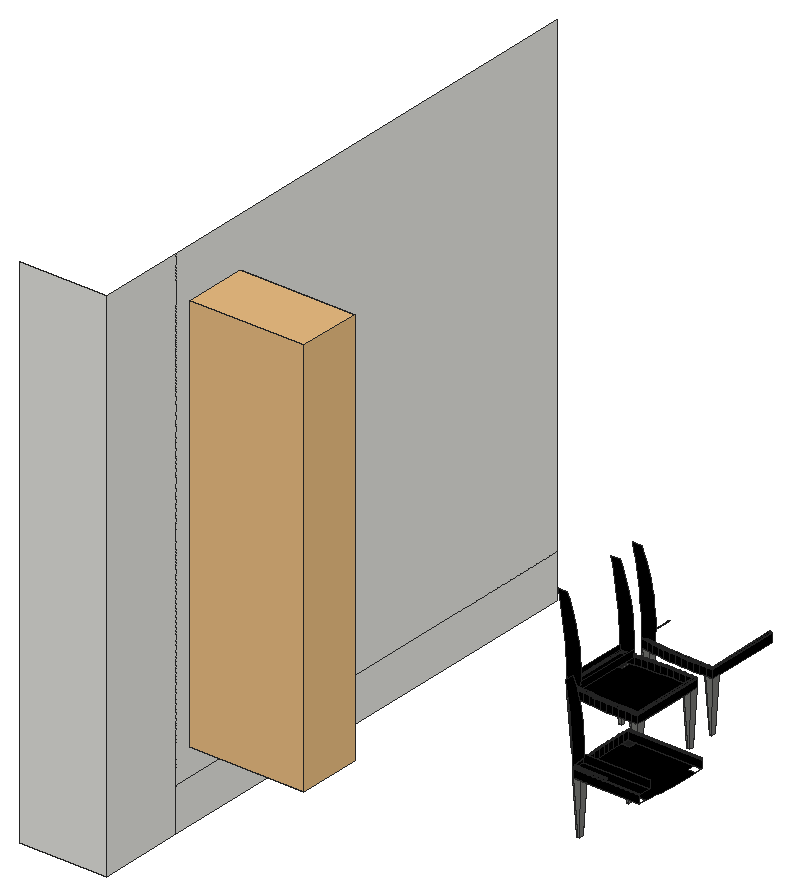
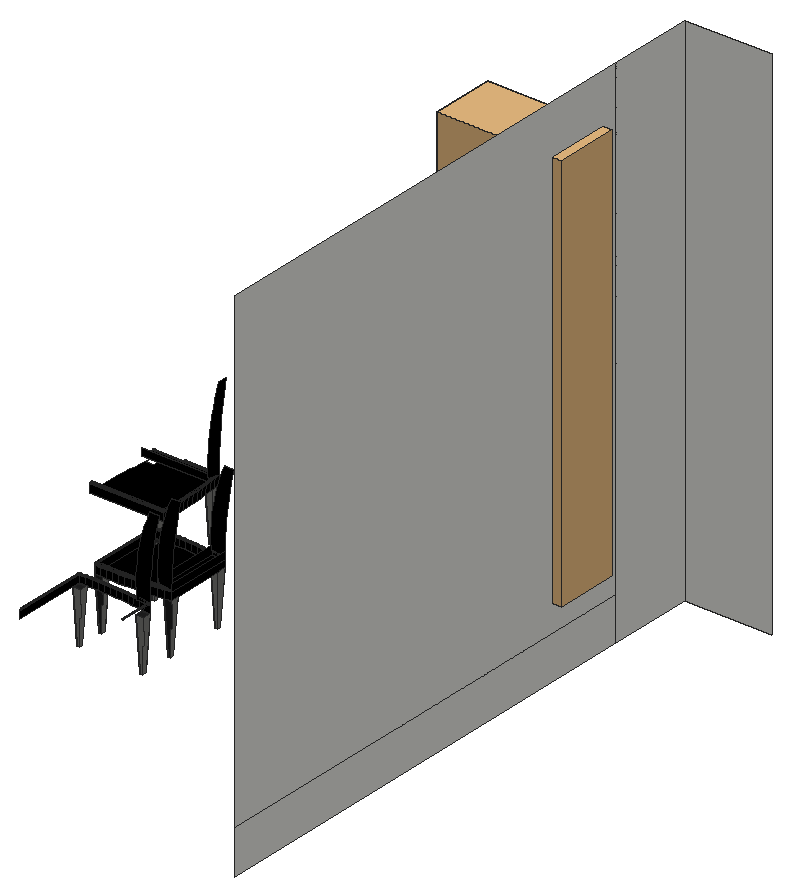
# SketchUp Ruby script. Lengths in inches.
U = 1.inch
M = Sketchup.active_model
def pt(a) = Geom::Point3d.new(a.map { |v| v * U })
def face(e, loops, mat)
  f = e.add_face(loops[0].map { |a| pt(a) })
  loops[1..].each { |l| e.add_face(l.map { |a| pt(a) }).erase! }
  f.material = f.back_material = mat if mat
  f
end
# faces: each face lists its corners as indices into pts; further lists are holes
def faces(e, pts, list, mat = nil) = list.each { |f| face(e, (f[0].is_a?(Array) ? f : [f]).map { |l| l.map { |i| pts[i] } }, mat) }
# xy, xz, yz: faces in a plane at the given z, y or x. An outline is a flat list of corners, or four numbers for a rectangle; further outlines are holes
def ring(l) = l.size == 4 ? [[l[0], l[1]], [l[2], l[1]], [l[2], l[3]], [l[0], l[3]]] : l.each_slice(2).to_a
def flat(e, list, mat, &to3) = list.each { |f| face(e, (f[0].is_a?(Array) ? f : [f]).map { |l| ring(l).map { |u, v| to3.(u, v) } }, mat) }
def xy(e, z, list, mat = nil) = flat(e, list, mat) { |x, y| [x, y, z] }
def xz(e, y, list, mat = nil) = flat(e, list, mat) { |x, z| [x, y, z] }
def yz(e, x, list, mat = nil) = flat(e, list, mat) { |y, z| [x, y, z] }
def lines(e, pts, list) = list.each { |a, b| e.add_line(pt(pts[a]), pt(pts[b])) }
# prism: a flat outline (further loops are holes) pulled along v
def prism(e, loops, v, mat = nil)
  f = face(e, loops, mat); d = Geom::Vector3d.new(v.map { |x| x * U })
  f.pushpull(f.normal.samedirection?(d) ? d.length : -d.length)
end
def box(e, o, s, mat = nil) = prism(e, [[o, [o[0] + s[0], o[1], o[2]], [o[0] + s[0], o[1] + s[1], o[2]], [o[0], o[1] + s[1], o[2]]]], [0, 0, s[2]], mat)
def at(x, y, z, deg = 0) = Geom::Transformation.translation(pt([x, y, z])) * Geom::Transformation.rotation(ORIGIN, Z_AXIS, deg.degrees)
def axes(o, x, y, z) = Geom::Transformation.new([*x, 0, *y, 0, *z, 0, *pt(o).to_a, 1])
def part(name) = M.definitions.add(name)
# library, detail: a bought-in or finely detailed component or shape, given as its bounding box
def library(name, o, s) = part(name).tap { |d| box(d.entities, o, s) }
def detail(e, o, s) = box(e.add_group.entities, o, s)
def put(e, d, t, mat = nil) = e.add_instance(d, t).tap { |i| i.material = mat if mat }
def group(e, t, mat = nil) = e.add_group.tap { |g| g.transformation = t; g.material = mat if mat }.entities
root = M.entities
M.materials.add("Color_008").color = [30, 30, 30]
M.materials.add("[Color M09]").color = [0, 0, 0]
M.materials.add("[Metal Seamed]").color = [118, 119, 115]
c1 = library("Group\#1",[0,0,0],[34.5,17.48,110.79])
xy(root,12,[[105.836,60.75,106.653,61.567],[104.815,79.026,105.632,79.843],[100.046,87.836,100.863,88.653],[81.769,88.857,82.586,89.674],[81.769,105.091,82.586,105.908],
  [100.046,106.112,100.863,106.929],[100.046,113.742,100.863,114.558],[81.769,114.763,82.586,115.58]],"Color_008")
xy(root,26.704,[[105.172,60.085,107.317,62.231],[104.151,78.362,106.296,80.507],[99.382,87.171,101.527,89.317],[81.105,88.193,83.25,90.338],[81.105,104.427,83.25,106.572],
  [99.382,105.448,101.527,107.593],[99.382,113.077,101.527,115.223],[81.105,114.098,83.25,116.244]],"Color_008")
xy(root,26.704,[[105.172,60.085,104.932,61.775,104.719,63.469,104.535,65.165,104.379,66.865,104.252,68.567,104.152,70.271,104.081,71.976,104.038,73.682,104.024,75.389,104.038,77.096,104.08,78.802,104.151,80.507,104.151,78.362,106.296,78.362,106.296,80.507,122.427,80.507,122.427,78.362,124.573,78.362,124.573,80.507,124.643,78.802,124.686,77.096,124.7,75.389,124.685,73.682,124.642,71.976,124.571,70.271,124.472,68.567,124.344,66.865,124.188,65.165,124.004,63.469,123.792,61.775,123.552,60.085,123.552,62.231,121.406,62.231,121.406,60.085,107.317,60.085,107.317,62.231,105.172,62.231],[96.409,87.045,94.702,87.059,92.996,87.102,91.291,87.173,89.587,87.272,87.885,87.4,86.185,87.556,84.488,87.74,82.795,87.952,81.105,88.193,83.25,88.193,83.25,90.338,81.105,90.338,81.105,104.427,83.25,104.427,83.25,106.572,81.105,106.572,82.795,106.8125,84.488,107.025,86.185,107.209,87.885,107.365,89.587,107.493,91.291,107.592,92.996,107.663,94.702,107.706,96.409,107.72,98.115,107.706,99.822,107.664,101.527,107.593,99.382,107.593,99.382,105.448,101.527,105.448,101.527,89.317,99.382,89.317,99.382,87.171,101.527,87.171,99.822,87.101,98.115,87.058]],"[Color M09]")
xy(root,28.845,[[105.172,60.085,123.552,63.622],[81.105,88.193,84.642,106.572]],"[Color M09]")
xz(root,0,[[0,0,24,144]])
xz(root,60.085,[[105.172,26.704,123.552,28.845]],"[Color M09]")
xz(root,80.507,[[104.151,26.704,124.573,28.845]],"[Color M09]")
xz(root,88.193,[[81.105,28.845,81.079,30.792,81.019,32.738,80.925,34.683,80.797,36.626,80.634,38.566,80.438,40.503,80.208,42.436,79.945,44.365,79.647,46.29,79.316,48.208,78.952,50.121,78.554,52.027,81.004,52.027,81.733,50.191,82.387,48.328,82.965,46.44,83.466,44.53,83.89,42.602,84.235,40.658,84.502,38.701,84.689,36.736,84.797,34.764,84.825,32.79,84.773,30.816,84.642,28.845]],"[Color M09]")
xz(root,106.572,[[81.105,28.845,84.642,28.845,84.773,30.816,84.825,32.79,84.797,34.764,84.689,36.736,84.502,38.701,84.235,40.658,83.89,42.602,83.466,44.53,82.965,46.44,82.387,48.328,81.733,50.191,81.004,52.027,78.554,52.027,78.952,50.121,79.316,48.208,79.647,46.29,79.945,44.365,80.208,42.436,80.438,40.503,80.634,38.566,80.797,36.626,80.925,34.683,81.019,32.738,81.079,30.792]],"[Color M09]")
xz(root,114.098,[[81.105,28.845,81.079,30.792,81.019,32.738,80.925,34.683,80.797,36.626,80.634,38.566,80.438,40.503,80.208,42.436,79.945,44.365,79.647,46.29,79.316,48.208,78.952,50.121,78.554,52.027,81.004,52.027,81.733,50.191,82.387,48.328,82.965,46.44,83.466,44.53,83.89,42.602,84.235,40.658,84.502,38.701,84.689,36.736,84.797,34.764,84.825,32.79,84.773,30.816,84.642,28.845]],"[Color M09]")
yz(root,24,[[0,0,24,144],[24,0,156,12],[24,12,156,144]])
yz(root,81.105,[[88.193,26.704,106.572,28.845]],"[Color M09]")
yz(root,101.527,[[87.171,26.704,107.593,28.845],[113.077,26.704,133.499,28.845]],"[Color M09]")
yz(root,105.172,[[60.085,28.845,63.622,28.845,63.754,30.816,63.806,32.79,63.777,34.764,63.67,36.736,63.482,38.701,63.216,40.658,62.87,42.602,62.446,44.53,61.945,46.44,61.367,48.328,60.713,50.191,59.985,52.027,57.534,52.027,57.932,50.121,58.297,48.208,58.628,46.29,58.925,44.365,59.189,42.436,59.419,40.503,59.615,38.566,59.777,36.626,59.905,34.683,59.999,32.738,60.059,30.792]],"[Color M09]")
p = [[106.653,60.75,12],[107.317,60.085,26.704],[105.172,60.085,26.704],[105.836,60.75,12],[105.172,62.231,26.704],[105.836,61.567,12],
  [106.653,61.567,12],[107.317,62.231,26.704],[105.632,79.026,12],[106.296,78.362,26.704],[104.151,78.362,26.704],[104.815,79.026,12],
  [104.151,80.507,26.704],[104.815,79.843,12],[105.632,79.843,12],[106.296,80.507,26.704],[100.863,87.836,12],[101.527,87.171,26.704],
  [99.382,87.171,26.704],[100.046,87.836,12],[99.382,89.317,26.704],[100.046,88.653,12],[100.863,88.653,12],[101.527,89.317,26.704],
  [82.586,88.857,12],[83.25,88.193,26.704],[81.105,88.193,26.704],[81.769,88.857,12],[81.105,90.338,26.704],[81.769,89.674,12],
  [82.586,89.674,12],[83.25,90.338,26.704],[82.586,105.091,12],[83.25,104.427,26.704],[81.105,104.427,26.704],[81.769,105.091,12],
  [81.105,106.572,26.704],[81.769,105.908,12],[82.586,105.908,12],[83.25,106.572,26.704],[100.863,106.112,12],[101.527,105.448,26.704],
  [99.382,105.448,26.704],[100.046,106.112,12],[99.382,107.593,26.704],[100.046,106.929,12],[100.863,106.929,12],[101.527,107.593,26.704],
  [100.863,113.742,12],[101.527,113.077,26.704],[99.382,113.077,26.704],[100.046,113.742,12],[99.382,115.223,26.704],[100.046,114.558,12],
  [100.863,114.558,12],[101.527,115.223,26.704],[82.586,114.763,12],[83.25,114.098,26.704],[81.105,114.098,26.704],[81.769,114.763,12],
  [81.105,116.244,26.704],[81.769,115.58,12],[82.586,115.58,12],[83.25,116.244,26.704],[104.932,61.775,28.845],[104.932,61.775,26.704],
  [105.172,60.085,28.845],[104.719,63.469,28.845],[104.719,63.469,26.704],[104.535,65.165,28.845],[104.535,65.165,26.704],[104.379,66.865,28.845],
  [104.379,66.865,26.704],[104.252,68.567,28.845],[104.252,68.567,26.704],[104.152,70.271,28.845],[104.152,70.271,26.704],[104.081,71.976,28.845],
  [104.081,71.976,26.704],[104.038,73.682,26.704],[104.038,73.682,28.845],[104.024,75.389,26.704],[104.024,75.389,28.845],[104.038,77.096,26.704],
  [104.038,77.096,28.845],[104.08,78.802,26.704],[104.08,78.802,28.845],[104.151,80.507,28.845],[94.702,87.059,26.704],[94.702,87.059,28.845],
  [96.409,87.045,28.845],[96.409,87.045,26.704],[98.115,87.058,28.845],[98.115,87.058,26.704],[92.996,87.102,26.704],[92.996,87.102,28.845],
  [91.291,87.173,28.845],[91.291,87.173,26.704],[99.822,87.101,28.845],[99.822,87.101,26.704],[101.527,87.171,28.845],[89.587,87.272,28.845],
  [89.587,87.272,26.704],[87.885,87.4,28.845],[87.885,87.4,26.704],[86.185,87.556,28.845],[86.185,87.556,26.704],[84.488,87.74,28.845],
  [84.488,87.74,26.704],[82.795,87.952,28.845],[82.795,87.952,26.704],[81.105,88.193,28.845],[82.795,106.8125,28.845],[82.795,106.8125,26.704],
  [81.105,106.572,28.845],[84.488,107.025,28.845],[84.488,107.025,26.704],[86.185,107.209,28.845],[86.185,107.209,26.704],[87.885,107.365,28.845],
  [87.885,107.365,26.704],[89.587,107.493,28.845],[89.587,107.493,26.704],[91.291,107.592,28.845],[91.291,107.592,26.704],[92.996,107.663,28.845],
  [92.996,107.663,26.704],[99.822,107.664,28.845],[99.822,107.664,26.704],[101.527,107.593,28.845],[94.702,107.706,26.704],[94.702,107.706,28.845],
  [96.409,107.72,26.704],[96.409,107.72,28.845],[98.115,107.706,26.704],[98.115,107.706,28.845],[92.996,113.008,26.704],[92.996,113.008,28.845],
  [91.291,113.079,28.845],[91.291,113.079,26.704],[94.702,112.965,28.845],[94.702,112.965,26.704],[96.409,112.95,28.845],[96.409,112.95,26.704],
  [98.115,112.964,28.845],[98.115,112.964,26.704],[99.822,113.007,28.845],[99.822,113.007,26.704],[101.527,113.077,28.845],[89.587,113.178,28.845],
  [89.587,113.178,26.704],[87.885,113.306,28.845],[87.885,113.306,26.704],[86.185,113.462,28.845],[86.185,113.462,26.704],[84.488,113.646,28.845],
  [84.488,113.646,26.704],[82.795,113.858,28.845],[82.795,113.858,26.704],[81.105,114.098,28.845],[104.941,61.777,28.992],[105.18,60.095,28.992],
  [123.552,60.085,28.845],[123.543,60.095,28.992],[104.729,63.47,28.992],[104.545,65.166,28.992],[105.172,63.754,30.816],[105.172,63.622,28.845],
  [123.552,63.622,28.845],[123.552,63.754,30.816],[104.389,66.866,28.992],[104.261,68.568,28.992],[104.162,70.271,28.992],[104.091,71.976,28.992],
  [104.048,73.683,28.992],[104.034,75.389,28.992],[104.048,77.096,28.992],[104.09,78.802,28.992],[104.16,80.498,28.992],[94.702,87.069,28.992],
  [96.409,87.054,28.992],[98.115,87.068,28.992],[92.996,87.111,28.992],[91.291,87.182,28.992],[99.821,87.11,28.992],[101.517,87.181,28.992],
  [89.587,87.282,28.992],[101.517,107.584,28.992],[87.886,87.409,28.992],[86.186,87.565,28.992],[84.489,87.749,28.992],[82.796,87.962,28.992],
  [81.115,88.201,28.992],[81.079,106.572,30.792],[81.079,88.193,30.792],[81.115,106.564,28.992],[84.773,106.572,30.816],[84.642,106.572,28.845],
  [84.642,88.193,28.845],[84.773,88.193,30.816],[82.796,106.803,28.992],[84.489,107.015,28.992],[86.186,107.199,28.992],[87.886,107.355,28.992],
  [89.587,107.483,28.992],[91.291,107.582,28.992],[92.996,107.653,28.992],[99.821,107.654,28.992],[94.702,107.696,28.992],[96.409,107.71,28.992],
  [98.115,107.697,28.992],[92.996,113.017,28.992],[91.291,113.088,28.992],[94.702,112.974,28.992],[96.409,112.96,28.992],[98.115,112.974,28.992],
  [99.821,113.016,28.992],[101.517,113.087,28.992],[89.587,113.1875,28.992],[101.517,133.49,28.992],[101.527,133.499,28.845],[87.886,113.315,28.992],
  [86.186,113.471,28.992],[84.489,113.655,28.992],[82.796,113.868,28.992],[81.115,114.107,28.992],[104.97,61.78,29.137],[105.205,60.124,29.137],
  [123.518,60.124,29.137],[114.362,60.124,29.137],[104.757,63.473,29.137],[104.573,65.169,29.137],[104.417,66.868,29.137],[104.29,68.57,29.137],
  [104.191,70.273,29.137],[104.119,71.978,29.137],[104.077,73.683,29.137],[104.0625,75.389,29.137],[104.076,77.095,29.137],[104.119,78.801,29.137],
  [104.188,80.469,29.137],[124.563,80.498,28.992],[124.536,80.469,29.137],[92.997,87.14,29.137],[91.292,87.211,29.137],[94.703,87.097,29.137],
  [96.409,87.083,29.137],[98.115,87.097,29.137],[99.82,87.139,29.137],[101.489,87.208,29.137],[89.589,87.31,29.137],[101.489,107.556,29.137],
  [87.888,87.438,29.137],[86.189,87.594,29.137],[84.493,87.778,29.137],[82.8,87.99,29.137],[81.143,88.226,29.137],[81.143,106.539,29.137],
  [81.143,97.382,29.137],[82.8,106.774,29.137],[84.493,106.987,29.137],[86.189,107.171,29.137],[87.888,107.327,29.137],[89.589,107.454,29.137],
  [91.292,107.554,29.137],[92.997,107.625,29.137],[94.703,107.667,29.137],[98.115,107.668,29.137],[99.82,107.626,29.137],[96.409,107.682,29.137],
  [92.997,113.046,29.137],[91.292,113.117,29.137],[94.703,113.003,29.137],[96.409,112.989,29.137],[98.115,113.003,29.137],[99.82,113.045,29.137],
  [101.489,113.114,29.137],[89.589,113.216,29.137],[101.489,133.462,29.137],[87.888,113.344,29.137],[86.189,113.5,29.137],[84.493,113.684,29.137],
  [82.8,113.896,29.137],[81.143,114.132,29.137],[105.017,61.787,29.276],[105.246,60.171,29.276],[114.362,60.171,29.276],[104.804,63.479,29.276],
  [104.62,65.174,29.276],[104.465,66.872,29.276],[104.337,68.573,29.276],[104.238,70.275,29.276],[104.167,71.98,29.276],[104.167,71.978,29.276],
  [104.124,73.684,29.276],[104.11,75.389,29.276],[104.124,77.094,29.276],[104.166,78.799,29.276],[104.233,80.422,29.276],[124.49,80.422,29.276],
  [92.999,87.187,29.276],[92.998,87.187,29.276],[91.295,87.258,29.276],[94.703,87.145,29.276],[96.409,87.13,29.276],[98.114,87.144,29.276],
  [99.819,87.186,29.276],[101.441,87.254,29.276],[89.592,87.358,29.276],[101.441,107.511,29.276],[87.892,87.485,29.276],[86.194,87.641,29.276],
  [84.498,87.825,29.276],[82.806,88.037,29.276],[81.191,88.267,29.276],[81.191,97.382,29.276],[81.191,106.498,29.276],[82.806,106.728,29.276],
  [84.498,106.94,29.276],[86.194,107.124,29.276],[87.892,107.279,29.276],[89.592,107.407,29.276],[91.295,107.506,29.276],[92.999,107.577,29.276],
  [92.998,107.577,29.276],[99.819,107.578,29.276],[94.703,107.62,29.276],[96.409,107.634,29.276],[98.114,107.62,29.276],[92.999,113.093,29.276],
  [92.998,113.093,29.276],[91.295,113.164,29.276],[94.703,113.05,29.276],[96.409,113.036,29.276],[98.114,113.05,29.276],[99.819,113.092,29.276],
  [101.441,113.16,29.276],[89.592,113.263,29.276],[101.441,133.417,29.276],[87.892,113.391,29.276],[86.194,113.547,29.276],[84.498,113.731,29.276],
  [82.806,113.943,29.276],[81.191,114.173,29.276],[81.191,123.288,29.276],[81.143,123.288,29.137],[105.081,61.795,29.408],[105.303,60.236,29.408],
  [114.362,60.236,29.408],[104.869,63.486,29.408],[104.685,65.181,29.408],[104.529,66.878,29.408],[104.402,68.577,29.408],[104.303,70.278,29.408],
  [104.232,71.98,29.408],[104.189,73.685,29.408],[104.232,71.982,29.408],[104.175,75.389,29.408],[104.189,77.093,29.408],[104.231,78.797,29.408],
  [104.296,80.356,29.408],[124.428,80.356,29.408],[93.002,87.252,29.408],[94.705,87.21,29.408],[96.409,87.195,29.408],[98.113,87.209,29.408],
  [99.817,87.251,29.408],[93,87.252,29.408],[91.298,87.323,29.408],[101.376,87.316,29.408],[89.597,87.423,29.408],[101.376,107.449,29.408],
  [87.897,87.55,29.408],[86.2,87.706,29.408],[84.506,87.89,29.408],[82.815,88.102,29.408],[81.256,88.323,29.408],[81.256,97.382,29.408],
  [81.256,106.441,29.408],[82.815,106.663,29.408],[84.506,106.875,29.408],[86.2,107.059,29.408],[87.897,107.215,29.408],[89.597,107.342,29.408],
  [91.298,107.441,29.408],[93,107.512,29.408],[99.817,107.513,29.408],[93.002,107.512,29.408],[94.705,107.555,29.408],[98.113,107.555,29.408],
  [96.409,107.569,29.408],[94.705,113.116,29.408],[96.409,113.101,29.408],[98.113,113.115,29.408],[93,113.158,29.408],[91.298,113.229,29.408],
  [93.002,113.158,29.408],[99.817,113.157,29.408],[101.376,113.222,29.408],[89.597,113.328,29.408],[101.376,133.354,29.408],[87.897,113.456,29.408],
  [86.2,113.612,29.408],[84.506,113.795,29.408],[82.815,114.007,29.408],[81.256,114.229,29.408],[81.256,123.288,29.408],[105.162,61.806,29.531],
  [105.374,60.318,29.531],[114.362,60.318,29.531],[104.95,63.496,29.531],[104.767,65.189,29.531],[104.611,66.884,29.531],[104.484,68.583,29.531],
  [104.384,70.283,29.531],[104.314,71.982,29.531],[104.313,71.986,29.531],[104.271,73.686,29.531],[104.257,75.389,29.531],[104.27,77.092,29.531],
  [104.313,78.794,29.531],[104.374,80.275,29.531],[124.35,80.275,29.531],[93.006,87.334,29.531],[94.706,87.291,29.531],[96.409,87.277,29.531],
  [98.112,87.291,29.531],[99.814,87.333,29.531],[91.302,87.405,29.531],[89.602,87.504,29.531],[93.002,87.334,29.531],[101.294,87.395,29.531],
  [101.294,107.37,29.531],[87.904,87.631,29.531],[86.208,87.787,29.531],[84.515,87.971,29.531],[82.826,88.183,29.531],[81.338,88.394,29.531],
  [81.338,97.382,29.531],[81.338,106.37,29.531],[82.826,106.582,29.531],[84.515,106.794,29.531],[86.208,106.978,29.531],[87.904,107.133,29.531],
  [89.602,107.261,29.531],[91.302,107.36,29.531],[93.002,107.431,29.531],[93.006,107.431,29.531],[94.706,107.473,29.531],[98.112,107.474,29.531],
  [99.814,107.431,29.531],[96.409,107.488,29.531],[93.006,113.24,29.531],[94.706,113.197,29.531],[96.409,113.183,29.531],[98.112,113.197,29.531],
  [99.814,113.239,29.531],[91.302,113.311,29.531],[89.602,113.41,29.531],[93.002,113.24,29.531],[101.294,113.3,29.531],[101.294,133.276,29.531],
  [87.904,113.537,29.531],[86.208,113.693,29.531],[84.515,113.877,29.531],[82.826,114.088,29.531],[81.338,114.3,29.531],[81.338,123.288,29.531],
  [105.258,61.819,29.641],[105.458,60.415,29.641],[114.362,60.415,29.641],[105.047,63.507,29.641],[104.481,70.287,29.641],[104.411,71.984,29.641],
  [104.41,71.99,29.641],[104.368,77.09,29.641],[104.41,78.791,29.641],[104.467,80.178,29.641],[124.256,80.178,29.641],[93.004,87.431,29.641],
  [91.307,87.502,29.641],[93.01,87.431,29.641],[94.708,87.388,29.641],[96.409,87.374,29.641],[98.11,87.388,29.641],[99.811,87.43,29.641],
  [101.197,87.488,29.641],[89.609,87.601,29.641],[101.197,107.277,29.641],[87.912,87.728,29.641],[86.218,87.884,29.641],[84.527,88.067,29.641],
  [82.839,88.279,29.641],[81.435,88.479,29.641],[81.435,97.382,29.641],[81.435,106.286,29.641],[82.839,106.486,29.641],[84.527,106.697,29.641],
  [86.218,106.881,29.641],[87.912,107.036,29.641],[89.609,107.164,29.641],[91.307,107.263,29.641],[93.004,107.333,29.641],[93.01,107.334,29.641],
  [94.708,107.376,29.641],[98.11,107.377,29.641],[99.811,107.334,29.641],[96.409,107.39,29.641]]
faces(root,p,[[0,1,2,3],[4,5,3,2],[6,7,1,0],[7,6,5,4],[8,9,10,11],[12,13,11,10],[14,15,9,8],[15,14,13,12],
  [16,17,18,19],[20,21,19,18],[22,23,17,16],[24,25,26,27],[28,29,27,26],[30,31,25,24],[23,22,21,20],[31,30,29,28],
  [32,33,34,35],[35,34,36,37],[33,32,38,39],[40,41,42,43],[43,42,44,45],[41,40,46,47],[48,49,50,51],[52,53,51,50],
  [54,55,49,48],[56,57,58,59],[60,61,59,58],[62,63,57,56],[55,54,53,52],[63,62,61,60]],"[Metal Seamed]")
faces(root,p,[[39,38,37,36],[47,46,45,44]],"Color_008")
faces(root,p,[[64,65,2,66],[67,68,65,64],[69,70,68,67],[71,72,70,69],[73,74,72,71],[75,76,74,73],[77,78,76,75],[77,78,79,80],
  [80,79,81,82],[82,81,83,84],[84,83,85,86],[86,85,12,87],[88,89,90,91],[91,90,92,93],[94,95,96,97],[94,95,89,88],
  [93,92,98,99],[99,98,100,17],[97,96,101,102],[102,101,103,104],[104,103,105,106],[106,105,107,108],[108,107,109,110],[110,109,111,26],
  [112,113,36,114],[115,116,113,112],[117,118,116,115],[119,120,118,117],[121,122,120,119],[123,124,122,121],[125,126,124,123],[127,128,47,129],
  [125,126,130,131],[131,130,132,133],[133,132,134,135],[135,134,128,127],[136,137,138,139],[136,137,140,141],[141,140,142,143],[143,142,144,145],
  [145,144,146,147],[147,146,148,49],[139,138,149,150],[150,149,151,152],[152,151,153,154],[154,153,155,156],[156,155,157,158],[158,157,159,58],
  [160,64,66,161],[161,66,162,163],[164,67,64,160],[165,69,67,164],[166,167,168,169],[170,71,69,165],[171,73,71,170],[172,75,73,171],
  [173,77,75,172],[173,77,80,174],[174,80,82,175],[175,82,84,176],[176,84,86,177],[177,86,87,178],[89,179,180,90],[90,180,181,92],
  [95,182,183,96],[95,182,179,89],[92,181,184,98],[98,184,185,100],[96,183,186,101],[187,129,100,185],[101,186,188,103],[103,188,189,105],
  [105,189,190,107],[107,190,191,109],[109,191,192,111],[114,193,194,111],[195,114,111,192],[196,197,198,199],[200,112,114,195],[201,115,112,200],
  [202,117,115,201],[203,119,117,202],[204,121,119,203],[205,123,121,204],[206,125,123,205],[207,127,129,187],[206,125,131,208],[208,131,133,209],
  [209,133,135,210],[210,135,127,207],[137,211,212,138],[137,211,213,140],[140,213,214,142],[142,214,215,144],[144,215,216,146],[146,216,217,148],
  [138,212,218,149],[219,220,148,217],[149,218,221,151],[151,221,222,153],[153,222,223,155],[155,223,224,157],[157,224,225,159],[226,160,161,227],
  [227,161,163,228,229],[230,164,160,226],[231,165,164,230],[232,170,165,231],[233,171,170,232],[234,172,171,233],[173,172,234,235],[235,173,174,236],
  [236,174,175,237],[237,175,176,238],[238,176,177,239],[239,177,178,240],[240,178,241,242],[183,182,243,244],[182,243,245,179],[179,245,246,180],
  [180,246,247,181],[181,247,248,184],[184,248,249,185],[183,244,250,186],[251,187,185,249],[186,250,252,188],[188,252,253,189],[189,253,254,190],
  [190,254,255,191],[191,255,256,192],[257,195,192,256,258],[259,200,195,257],[260,201,200,259],[261,202,201,260],[262,203,202,261],[263,204,203,262],
  [264,205,204,263],[206,205,264,265],[265,206,208,266],[267,210,207,268],[268,207,187,251],[266,208,209,269],[269,209,210,267],[212,211,270,271],
  [211,270,272,213],[213,272,273,214],[214,273,274,215],[215,274,275,216],[216,275,276,217],[212,271,277,218],[278,219,217,276],[218,277,279,221],
  [221,279,280,222],[222,280,281,223],[223,281,282,224],[224,282,283,225],[284,226,227,285],[285,227,229,286],[287,230,226,284],[288,231,230,287],
  [289,232,231,288],[290,233,232,289],[291,234,233,290],[292,235,234,291,293],[235,236,294,292],[294,236,237,295],[295,237,238,296],[296,238,239,297],
  [297,239,240,298],[298,240,242,299],[243,300,301,302,244],[245,243,300,303],[245,303,304,246],[246,304,305,247],[247,305,306,248],[248,306,307,249],
  [244,302,308,250],[309,251,249,307],[250,308,310,252],[252,310,311,253],[253,311,312,254],[254,312,313,255],[255,313,314,256],[256,314,315,258],
  [316,257,258,315],[317,259,257,316],[318,260,259,317],[319,261,260,318],[320,262,261,319],[321,263,262,320],[322,264,263,321],[323,265,264,322,324],
  [325,268,251,309],[265,266,326,323],[326,266,269,327],[327,269,267,328],[328,267,268,325],[270,329,330,331,271],[272,270,329,332],[272,332,333,273],
  [273,333,334,274],[274,334,335,275],[275,335,336,276],[271,331,337,277],[338,278,276,336],[277,337,339,279],[279,339,340,280],[280,340,341,281],
  [281,341,342,282],[282,342,343,283],[283,343,344,345],[346,284,285,347],[347,285,286,348],[349,287,284,346],[350,288,287,349],[351,289,288,350],
  [352,290,289,351],[353,291,290,352],[293,291,353,354],[292,294,355,356],[354,356,292,293],[355,294,295,357],[357,295,296,358],[358,296,297,359],
  [359,297,298,360],[360,298,299,361],[303,300,362,363],[303,363,364,304],[304,364,365,305],[305,365,366,306],[302,301,367,368],[367,362,300,301],
  [306,366,369,307],[302,368,370,308],[371,309,307,369],[308,370,372,310],[310,372,373,311],[311,373,374,312],[312,374,375,313],[313,375,376,314],
  [314,376,377,315],[378,316,315,377],[379,317,316,378],[380,318,317,379],[381,319,318,380],[382,320,319,381],[383,321,320,382],[384,322,321,383],
  [324,322,384,385],[386,325,309,371],[385,387,323,324],[323,326,388,387],[389,328,325,386],[388,326,327,390],[390,327,328,389],[332,391,392,333],
  [333,392,393,334],[331,330,394,395],[332,329,396,391],[394,396,329,330],[334,393,397,335],[335,397,398,336],[331,395,399,337],[400,338,336,398],
  [337,399,401,339],[339,401,402,340],[340,402,403,341],[341,403,404,342],[342,404,405,343],[343,405,406,344],[407,346,347,408],[408,347,348,409],
  [410,349,346,407],[411,350,349,410],[412,351,350,411],[413,352,351,412],[414,353,352,413],[354,353,414,415],[416,415,354,356],[356,355,417,416],
  [417,355,357,418],[418,357,358,419],[419,358,359,420],[420,359,360,421],[421,360,361,422],[363,362,423,424],[363,424,425,364],[364,425,426,365],
  [365,426,427,366],[368,428,429,370],[368,367,430,428],[423,430,367,362],[366,427,431,369],[432,371,369,431],[370,429,433,372],[372,433,434,373],
  [373,434,435,374],[374,435,436,375],[375,436,437,376],[376,437,438,377],[439,378,377,438],[440,379,378,439],[441,380,379,440],[442,381,380,441],
  [443,382,381,442],[444,383,382,443],[445,384,383,444],[385,384,445,446],[447,446,385,387],[387,388,448,447],[449,389,386,450],[450,386,371,432],
  [448,388,390,451],[451,390,389,449],[391,396,452,453],[391,453,454,392],[392,454,455,393],[393,455,456,397],[395,457,458,399],[395,394,459,457],
  [452,459,394,396],[397,456,460,398],[461,400,398,460],[399,458,462,401],[401,462,463,402],[402,463,464,403],[403,464,465,404],[404,465,466,405],
  [405,466,467,406],[468,407,408,469],[469,408,409,470],[471,410,407,468],[415,414,472,473],[473,474,416,415],[475,419,420,476],[477,421,422,478],
  [428,430,479,480],[424,423,481,482],[479,481,423,430],[424,482,483,425],[425,483,484,426],[426,484,485,427],[427,485,486,431],[428,480,487,429],
  [488,432,431,486],[429,487,489,433],[433,489,490,434],[434,490,491,435],[435,491,492,436],[436,492,493,437],[437,493,494,438],[495,439,438,494],
  [496,440,439,495],[497,441,440,496],[498,442,441,497],[499,443,442,498],[500,444,443,499],[501,445,444,500],[446,445,501,502],[502,503,447,446],
  [447,448,504,503],[505,449,450,506],[506,450,432,488],[504,448,451,507],[507,451,449,505]],"[Color M09]")
put(root,c1,at(21.32,28.64,19.625))
